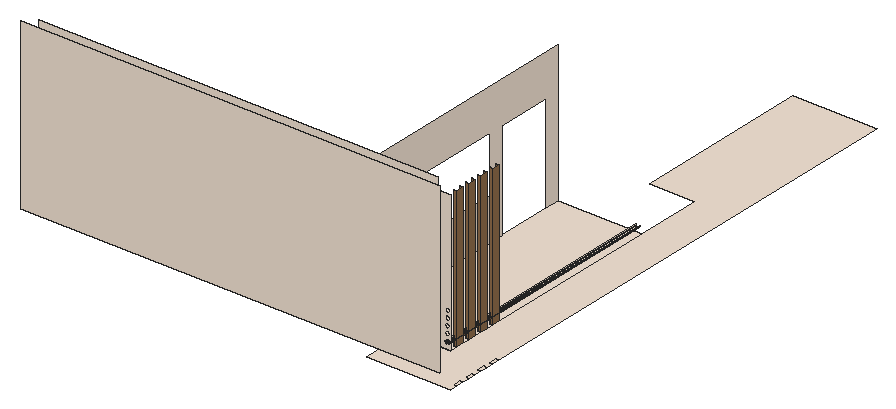
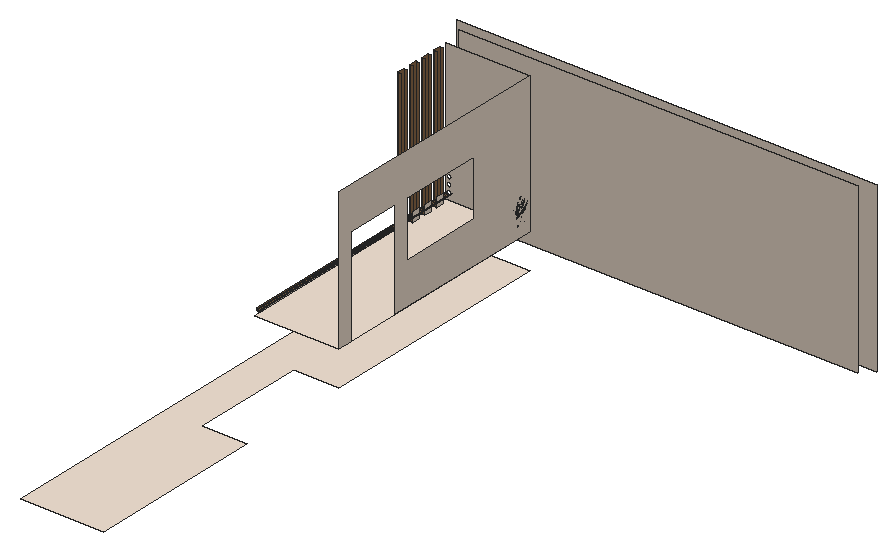
# SketchUp Ruby script. Lengths in inches.
U = 1.inch
M = Sketchup.active_model
def pt(a) = Geom::Point3d.new(a.map { |v| v * U })
def face(e, loops, mat)
  f = e.add_face(loops[0].map { |a| pt(a) })
  loops[1..].each { |l| e.add_face(l.map { |a| pt(a) }).erase! }
  f.material = f.back_material = mat if mat
  f
end
# faces: each face lists its corners as indices into pts; further lists are holes
def faces(e, pts, list, mat = nil) = list.each { |f| face(e, (f[0].is_a?(Array) ? f : [f]).map { |l| l.map { |i| pts[i] } }, mat) }
# xy, xz, yz: faces in a plane at the given z, y or x. An outline is a flat list of corners, or four numbers for a rectangle; further outlines are holes
def ring(l) = l.size == 4 ? [[l[0], l[1]], [l[2], l[1]], [l[2], l[3]], [l[0], l[3]]] : l.each_slice(2).to_a
def flat(e, list, mat, &to3) = list.each { |f| face(e, (f[0].is_a?(Array) ? f : [f]).map { |l| ring(l).map { |u, v| to3.(u, v) } }, mat) }
def xy(e, z, list, mat = nil) = flat(e, list, mat) { |x, y| [x, y, z] }
def xz(e, y, list, mat = nil) = flat(e, list, mat) { |x, z| [x, y, z] }
def yz(e, x, list, mat = nil) = flat(e, list, mat) { |y, z| [x, y, z] }
def lines(e, pts, list) = list.each { |a, b| e.add_line(pt(pts[a]), pt(pts[b])) }
# prism: a flat outline (further loops are holes) pulled along v
def prism(e, loops, v, mat = nil)
  f = face(e, loops, mat); d = Geom::Vector3d.new(v.map { |x| x * U })
  f.pushpull(f.normal.samedirection?(d) ? d.length : -d.length)
end
def box(e, o, s, mat = nil) = prism(e, [[o, [o[0] + s[0], o[1], o[2]], [o[0] + s[0], o[1] + s[1], o[2]], [o[0], o[1] + s[1], o[2]]]], [0, 0, s[2]], mat)
def at(x, y, z, deg = 0) = Geom::Transformation.translation(pt([x, y, z])) * Geom::Transformation.rotation(ORIGIN, Z_AXIS, deg.degrees)
def axes(o, x, y, z) = Geom::Transformation.new([*x, 0, *y, 0, *z, 0, *pt(o).to_a, 1])
def part(name) = M.definitions.add(name)
# library, detail: a bought-in or finely detailed component or shape, given as its bounding box
def library(name, o, s) = part(name).tap { |d| box(d.entities, o, s) }
def detail(e, o, s) = box(e.add_group.entities, o, s)
def put(e, d, t, mat = nil) = e.add_instance(d, t).tap { |i| i.material = mat if mat }
def group(e, t, mat = nil) = e.add_group.tap { |g| g.transformation = t; g.material = mat if mat }.entities
root = M.entities
M.materials.add("C01_Vanilla_Cream").color = [244, 228, 212]
M.materials.add("LightPink_Translucent").color = [144, 107, 117]
M.materials["LightPink_Translucent"].alpha = 0.75
M.materials.add("Wood_Floor_01_1K").color = [146, 111, 76]
c1 = part("blade")
p = [[2.15,0.21,22],[0,0.17,0],[0.09,0.45,0],[2.18,0.31,22],[2.29,0.31,22],[0.38,0.45,0],
  [2.48,0.24,33],[2.49,0.24,33],[2.48,0.22,33]]
faces(c1.entities,p,[[0,1,2,3],[4,5,2,3],[6,3,4,7],[8,0,3,6]])
c2 = part("seeds")
p = [[0.3,-0.1,1.38],[-0.01,-0.03,1.59],[-0.01,-0.03,0.03],[0.14,-0.07,-0.07],[0.29,-0.03,3],[0.15,0.01,3.11]]
faces(c2.entities,p,[[0,1,2,3],[1,0,4,5]],"LightPink_Translucent")
c3 = part("blade with seeds")
put(c3.entities,c1,at(0,0,0))
put(c3.entities,c2,axes([2.4,0.25,30.99],[1.5799,-0.05474,1.17369],[-0.12525,1.92788,0.29478],[-0.07173,-0.02425,1.56792]))
xy(root,132,[[288,12,288,216,326.85,216,326.85,314.71,288,314.71,288,468,360,468,360,63.65,357,63.65,357,57.2,360,57.2,360,50.74,357,50.74,357,44.28,360,44.28,360,37.83,357,37.83,357,31.37,360,31.37,360,24.91,357,24.91,357,18.46,360,18.46,360,12],[357,18.46,360,24.91],[357,31.37,360,37.83],[357,44.28,360,50.74],[357,57.2,360,63.65]],"C01_Vanilla_Cream")
xy(root,162,[[288,12,360,12,360,18.46,357,18.46,357,24.91,360,24.91,360,31.37,357,31.37,357,37.83,360,37.83,360,44.28,357,44.28,357,50.74,360,50.74,360,57.2,357,57.2,357,63.65,360,63.65,360,216,288,216],[357,18.46,360,24.91],[357,31.37,360,37.83],[357,44.28,360,50.74],[357,57.2,360,63.65]],"C01_Vanilla_Cream")
xz(root,0,[[0,150,360,294]],"C01_Vanilla_Cream")
xz(root,9,[[9,150,351,294]],"C01_Vanilla_Cream")
xz(root,12,[[[288,162,360,282],[357,184,357.52,184.07,358,184.27,358.41,184.59,358.73,185,358.93,185.48,359,186,358.93,186.52,358.73,187,358.41,187.41,358,187.73,357.52,187.93,357,188,356.48,187.93,356,187.73,355.59,187.41,355.27,187,355.07,186.52,355,186,355.07,185.48,355.27,185,355.59,184.59,356,184.27,356.48,184.07],[357,190,357.52,190.07,358,190.27,358.41,190.59,358.73,191,358.93,191.48,359,192,358.93,192.52,358.73,193,358.41,193.41,358,193.73,357.52,193.93,357,194,356.48,193.93,356,193.73,355.59,193.41,355.27,193,355.07,192.52,355,192,355.07,191.48,355.27,191,355.59,190.59,356,190.27,356.48,190.07],[357,178,357.52,178.07,358,178.27,358.41,178.59,358.73,179,358.93,179.48,359,180,358.93,180.52,358.73,181,358.41,181.41,358,181.73,357.52,181.93,357,182,356.48,181.93,356,181.73,355.59,181.41,355.27,181,355.07,180.52,355,180,355.07,179.48,355.27,179,355.59,178.59,356,178.27,356.48,178.07],[357,172,357.52,172.07,358,172.27,358.41,172.59,358.73,173,358.93,173.48,359,174,358.93,174.52,358.73,175,358.41,175.41,358,175.73,357.52,175.93,357,176,356.48,175.93,356,175.73,355.59,175.41,355.27,175,355.07,174.52,355,174,355.07,173.48,355.27,173,355.59,172.59,356,172.27,356.48,172.07],[357,166,357.52,166.07,358,166.27,358.41,166.59,358.73,167,358.93,167.48,359,168,358.93,168.52,358.73,169,358.41,169.41,358,169.73,357.52,169.93,357,170,356.48,169.93,356,169.73,355.59,169.41,355.27,169,355.07,168.52,355,168,355.07,167.48,355.27,167,355.59,166.59,356,166.27,356.48,166.07]]],"C01_Vanilla_Cream")
xz(root,18.46,[[357,162,360,282]],"Wood_Floor_01_1K")
xz(root,24.91,[[357,162,360,282]],"Wood_Floor_01_1K")
xz(root,31.37,[[357,162,360,282]],"Wood_Floor_01_1K")
xz(root,37.83,[[357,162,360,282]],"Wood_Floor_01_1K")
xz(root,44.28,[[357,162,360,282]],"Wood_Floor_01_1K")
xz(root,50.74,[[357,162,360,282]],"Wood_Floor_01_1K")
xz(root,57.2,[[357,162,360,282]],"Wood_Floor_01_1K")
xz(root,63.65,[[357,162,360,282]],"Wood_Floor_01_1K")
yz(root,288,[[[12,162,156,162,156,246,204,246,204,162,216,162,216,282,12,282],[72,198,144,246]]],"C01_Vanilla_Cream")
yz(root,357,[[18.46,162,24.91,166],[31.37,162,37.83,166],[44.28,162,50.74,166],[57.2,162,63.65,166],[18.46,166,24.91,170],
  [31.37,166,37.83,170],[44.28,166,50.74,170],[57.2,166,63.65,170]],"C01_Vanilla_Cream")
yz(root,360,[[18.46,162,24.91,282],[31.37,162,37.83,282],[44.28,162,50.74,282],[57.2,162,63.65,282]],"Wood_Floor_01_1K")
p = [[356.48,216,166.07],[357,216,166],[357,63.65,166],[357,57.2,166],[357,50.74,166],[357,44.28,166],
  [357,37.83,166],[357,31.37,166],[357,24.91,166],[357,18.46,166],[357,12,166],[356.48,12,166.07],
  [357.52,216,166.07],[357.52,12,166.07],[356,216,166.27],[356,12,166.27],[358,216,166.27],[358,12,166.27],
  [355.59,216,166.59],[355.59,12,166.59],[358.41,216,166.59],[358.41,12,166.59],[355.27,216,167],[355.27,12,167],
  [358.73,216,167],[358.73,12,167],[355.07,216,167.48],[355.07,12,167.48],[358.93,216,167.48],[358.93,12,167.48],
  [355,216,168],[355,12,168],[359,216,168],[359,12,168]]
faces(root,p,[[0,1,2,3,4,5,6,7,8,9,10,11],[14,0,11,15],[18,14,15,19],[22,18,19,23],[26,22,23,27],[30,26,27,31]],"C01_Vanilla_Cream")
faces(root,p,[[1,12,13,10,9,8,7,6,5,4,3,2],[12,16,17,13],[16,20,21,17],[20,24,25,21],[24,28,29,25],[28,32,33,29]],"Wood_Floor_01_1K")
put(root,c3,axes([295.875,21,164.91],[0.12726,0.15818,1.28532],[-0.58807,0.13317,0.10393],[-0.13291,-0.24832,0.54946]))
put(root,c3,axes([296.85,19.95,165.54],[-0.08515,-0.06907,1.31208],[-0.56828,0.04379,-0.2075],[-0.0907,-0.16522,0.10523]))
put(root,c3,axes([298.17,20.77,163.94],[-0.15825,0.09972,1.07251],[-0.47395,-0.17454,-0.23066],[0.08785,-0.21706,0.45856]))
put(root,c3,axes([297.44,21.12,165.74],[-0.26572,-0.40059,-0.53284],[0.54698,-0.22325,0.0643],[-0.06214,-0.19355,0.75375]))
put(root,c3,axes([295.72,20.58,163.94],[-0.03371,0.16116,1.07251],[-0.49286,0.13491,-0.23066],[-0.11521,-0.20831,0.45856]))
put(root,c3,axes([296.99,20.23,163.12],[-0.09338,0.01775,1.32257],[-0.51641,-0.1998,-0.20205],[0.00867,-0.16666,0.22528]))
put(root,c3,axes([298.55,21.51,165.74],[0.01449,-0.45571,-0.53284],[0.61002,0.03061,0.0643],[0.06438,-0.19306,0.75375]))
put(root,c3,axes([299.4,20.8,165.54],[-0.00537,-0.09805,1.31208],[-0.45391,-0.28338,-0.2075],[0.07018,-0.17178,0.10523]))
put(root,c3,axes([297.49,20.78,165.39],[0.16784,-0.37886,-0.2656],[0.48968,0.1105,0.3429],[-0.0449,-0.15254,0.65611]))
put(root,c3,axes([297.86,21.28,164.91],[-0.10366,0.16934,1.28532],[-0.43488,-0.35044,0.10393],[0.19618,-0.21841,0.54946]))
put(root,c3,axes([299.28,20.44,165.53],[-0.05654,0.03763,1.33037],[-0.55396,-0.12696,-0.12571],[-0.02005,-0.16422,0.23543]))
put(root,c3,axes([297.24,21.04,165.51],[-0.54728,-0.1235,-0.38324],[0.18759,-0.42344,-0.29685],[-0.05018,-0.17048,0.7333]))
put(root,c3,axes([297.58,19.98,164.07],[0.07142,0.28728,0.86145],[-0.3962,-0.15911,0.63294],[0.04263,-0.1471,0.18974]))
put(root,c3,axes([298.43,21.36,165.51],[-0.39855,-0.33102,-0.38324],[0.42102,-0.2899,-0.29685],[0.06064,-0.16819,0.7333]))
put(root,c3,axes([296.26,19.72,165.53],[-0.01039,0.05905,1.33037],[-0.51226,0.21431,-0.12571],[-0.15074,-0.10955,0.23543]))
put(root,c3,axes([296.15,20.77,165.82],[0.62019,-0.12663,0.40322],[0.10763,0.49673,0.33247],[-0.14586,-0.1464,0.83437]))
put(root,c3,axes([297.55,20.86,165.55],[0.54859,0.1288,0.36002],[-0.18759,0.42344,0.29685],[-0.03297,-0.16652,0.74497]))
put(root,c3,axes([297.71,21.02,165.78],[-0.54481,0.22937,-0.0912],[-0.26773,-0.4071,-0.50621],[-0.07188,-0.17155,0.76918]))
put(root,c3,axes([298.84,21.53,165.78],[-0.61188,-0.02441,-0.0912],[0.01672,-0.46217,-0.50621],[0.0425,-0.178,0.76918]))
put(root,c3,axes([298.8,21.23,165.39],[0.3767,-0.25939,-0.2656],[0.3566,0.29618,0.3429],[0.05426,-0.15048,0.65611]))
put(root,c3,axes([295.55,20.32,164.07],[0.29042,0.17147,0.86145],[-0.42295,0.10307,0.63294],[-0.0905,-0.13178,0.18974]))
put(root,c3,axes([297.7,20.83,165.55],[0.41024,-0.16744,0.04823],[0.2008,0.30532,0.37966],[-0.03962,-0.13459,0.57892]))
put(root,c3,axes([296.25,21.23,165.74],[-0.47473,-0.23813,-0.53284],[0.33738,-0.41728,0.0643],[-0.172,-0.14218,0.75375]))
put(root,c3,axes([296.08,20.91,165.39],[-0.08599,-0.39682,-0.2656],[0.49155,-0.10478,0.3429],[-0.13203,-0.11372,0.65611]))
put(root,c3,axes([296.29,20.88,165.55],[0.25304,-0.31296,0.04823],[0.36033,0.18221,0.37966],[-0.11649,-0.10034,0.57892]))
put(root,c3,axes([295.32,20.84,163.12],[-0.05393,0.0649,1.32257],[-0.545,0.13993,-0.20205],[-0.13166,-0.12729,0.22528]))
put(root,c3,axes([296.22,22.62,163.57],[-0.22864,-0.5052,-0.52377],[0.65862,-0.18195,-0.13747],[-0.02527,-0.17107,1.15612]))
put(root,c3,axes([295.02,21.49,164.91],[0.2068,0.08488,1.28532],[-0.42797,0.35609,0.10393],[-0.26673,-0.16064,0.54946]))
put(root,c3,axes([299.27,21.08,163.12],[-0.08333,-0.03881,1.32257],[-0.21404,-0.4336,-0.20205],[0.14439,-0.11767,0.22528]))
put(root,c3,axes([297.55,21.17,165.79],[-0.16784,0.37886,0.2656],[-0.48968,-0.1105,-0.3429],[-0.0449,-0.15254,0.65611]))
put(root,c3,axes([296.02,21.24,165.51],[-0.54938,0.11711,-0.38324],[-0.0961,-0.44351,-0.29685],[-0.14756,-0.1271,0.7333]))
put(root,c3,axes([298.8,21.33,165.55],[0.39645,0.33614,0.36002],[-0.42102,0.2899,0.29685],[0.07313,-0.15771,0.74497]))
put(root,c3,axes([296.41,20.85,166.07],[-0.37157,0.4723,-0.10215],[-0.5381,-0.2721,-0.56695],[-0.18705,-0.13344,0.86148]))
put(root,c3,axes([298.95,21.37,165.55],[0.45752,0.02296,0.04823],[-0.01254,0.34663,0.37966],[0.04787,-0.13278,0.57892]))
put(root,c3,axes([298.6,21.6,165.79],[-0.3767,0.25939,0.2656],[-0.3566,-0.29618,-0.3429],[0.05426,-0.15048,0.65611]))
put(root,c3,axes([299.27,22.3,165.74],[0.29081,-0.38873,-0.53284],[0.5096,0.27626,0.0643],[0.17364,-0.14084,0.75375]))
put(root,c3,axes([296.125,21.17,163.78],[-0.34808,-0.49367,0],[0.58235,-0.27531,-0.38706],[0.13264,-0.0627,1.22783]))
put(root,c3,axes([299.25,22.12,165.51],[-0.14302,-0.44985,-0.38324],[0.54163,-0.07869,-0.29685],[0.15522,-0.12083,0.7333]))
put(root,c3,axes([296.89,20.57,163.6],[-0.38473,0.28263,-0.02919],[-0.35252,-0.30954,-0.13237],[-0.02482,-0.08771,0.43661]))
put(root,c3,axes([294.98,20.71,165.54],[-0.11979,-0.00348,1.31208],[-0.38137,0.34775,-0.2075],[-0.20349,-0.07106,0.10523]))
put(root,c3,axes([299.51,22.44,165.78],[-0.515,-0.27165,-0.0912],[0.2967,-0.3934,-0.50621],[0.1455,-0.13675,0.76918]))
put(root,c3,axes([297.38,23.92,164.49],[0.48111,0.19866,1.13446],[-0.47133,0.42798,0.44862],[-0.21112,-0.25366,0.95105]))
put(root,c3,axes([296.37,21.24,165.79],[0.08599,0.39682,0.2656],[-0.49155,0.10478,-0.3429],[-0.13203,-0.11372,0.65611]))
put(root,c3,axes([294.87,22.55,163.51],[0,-0.49266,-0.37238],[0.62289,0,0],[0,-0.11221,1.18128]))
put(root,c3,axes([296.6,21.09,163.51],[0.52105,-0.24633,-0.37238],[0.31144,0.44171,0],[0.11867,-0.0561,1.18128]))
put(root,c3,axes([299.69,21.94,163.94],[-0.19889,-0.01459,1.07251],[-0.20376,-0.39145,-0.23066],[0.24434,-0.11074,0.45856]))
put(root,c3,axes([294.9,21.5,165.82],[0.45978,-0.36358,0.40322],[0.39653,0.38611,0.33247],[-0.21571,-0.06707,0.83437]))
put(root,c3,axes([300.78,22.32,165.53],[-0.07272,-0.00374,1.33037],[-0.30197,-0.40092,-0.12571],[0.12127,-0.13182,0.23543]))
put(root,c3,axes([297.22,22.1,163.54],[0.375,-0.3703,-0.46765],[0.46584,0.33578,-0.12274],[0.15027,-0.09237,1.03225]))
put(root,c3,axes([299.92,21.22,164.07],[-0.18544,0.25079,0.86145],[-0.15939,-0.33694,0.63294],[0.15316,-0.08443,0.18974]))
put(root,c3,axes([299.65,22.17,165.39],[0.48462,-0.07041,-0.2656],[0.12797,0.4025,0.3429],[0.13888,-0.10811,0.65611]))
put(root,c3,axes([295.11,21.49,165.55],[0.02803,-0.37463,0.04823],[0.42332,0.01027,0.37966],[-0.16216,-0.0392,0.57892]))
put(root,c3,axes([296.5625,22.75,163.66],[0.27012,-0.44393,-0.33554],[0.56127,0.21365,0.16149],[0,-0.10233,1.07733]))
put(root,c3,axes([294.94,21.61,165.39],[-0.31678,-0.30846,-0.2656],[0.36171,-0.29199,0.3429],[-0.18378,-0.04443,0.65611]))
put(root,c3,axes([296.81,22.53,164],[-0.06488,-0.56215,-0.21822],[0.6757,-0.03399,-0.37502],[0.11898,-0.07488,1.19781]))
put(root,c3,axes([295.13,22.5625,163.52],[0.38863,-0.30738,-0.23233],[0.38863,0.30738,0.23233],[0,-0.09901,1.0423]))
put(root,c3,axes([294.98,21.09,163.6],[-0.1606,0.40228,-0.02919],[-0.4943,-0.12375,-0.13237],[-0.07505,-0.0658,0.43661]))
put(root,c3,axes([299.26,22.4,165.79],[-0.48462,0.07041,0.2656],[-0.12797,-0.4025,-0.3429],[0.13888,-0.10811,0.65611]))
put(root,c3,axes([296.5,23.12,164],[-0.62699,-0.23507,-0.21822],[0.3019,-0.49615,-0.37502],[-0.0197,-0.12182,1.19781]))
put(root,c3,axes([294.71,22.92,163.78],[-0.69617,0,0],[0,-0.55062,-0.38706],[0,-0.12541,1.22783]))
put(root,c3,axes([294.83,21.94,163.94],[0.1087,0.13716,1.07251],[-0.25048,0.37284,-0.23066],[-0.25719,-0.08912,0.45856]))
put(root,c3,axes([296.72,21.29,163.52],[0.51941,0.1219,-0.23233],[-0.13078,0.42928,0.23233],[0.10471,-0.0495,1.0423]))
put(root,c3,axes([295.28,21.82,165.74],[-0.55654,-0.01186,-0.53284],[0.03738,-0.49951,0.0643],[-0.23578,-0.05271,0.75375]))
put(root,c3,axes([299.7,22.34,165.55],[0.3822,0.20719,0.04823],[-0.22252,0.29505,0.37966],[0.12254,-0.09539,0.57892]))
put(root,c3,axes([299.59,22.25,165.55],[0.13808,0.45342,0.36002],[-0.54163,0.07869,0.29685],[0.15963,-0.10664,0.74497]))
put(root,c3,axes([301.05,22.8,165.54],[0.07726,-0.07504,1.31208],[-0.09888,-0.46032,-0.2075],[0.19384,-0.08728,0.10523]))
put(root,c3,axes([295.25,22.78,163.75],[-0.51786,0.4142,0.23067],[-0.51817,-0.40984,-0.27369],[-0.01808,-0.11762,1.23664]))
put(root,c3,axes([294.52,21,165.53],[0.04127,0.04917,1.33037],[-0.19898,0.44196,-0.12571],[-0.20151,0.0032,0.23543]))
put(root,c3,axes([296.9,22.97,163.82],[0.6273,0.23878,0.18048],[-0.3019,0.49615,0.37502],[0,-0.11437,1.20407]))
put(root,c3,axes([296.65,23.64,163.83],[0.14756,-0.58378,-0.17572],[0.69966,0.10176,0.38453],[-0.12225,-0.08062,1.1733]))
put(root,c3,axes([295.09,21.92,165.51],[-0.40426,0.32635,-0.38324],[-0.35404,-0.34474,-0.29685],[-0.2054,-0.04965,0.7333]))
put(root,c3,axes([295.39,21.77,165.79],[0.31678,0.30846,0.2656],[-0.36171,0.29199,-0.3429],[-0.18378,-0.04443,0.65611]))
put(root,c3,axes([294.18,22.35,164.07],[0.35544,-0.03525,0.86145],[-0.22547,0.31061,0.63294],[-0.17565,-0.04659,0.18974]))
put(root,c3,axes([296.7,22.64,164.04],[-0.60457,0.03041,0.33554],[-0.05467,-0.50484,-0.16149],[0.10823,-0.05117,1.07733]))
put(root,c3,axes([295.31,21.58,165.78],[-0.02981,0.50103,-0.0912],[-0.56442,-0.01369,-0.50621],[-0.21738,-0.0348,0.76918]))
put(root,c3,axes([295.13,23.01,163.86],[0,0.49266,0.37238],[-0.62289,0,0],[0,-0.11221,1.18128]))
put(root,c3,axes([299.53,23.5,165.78],[-0.28012,-0.44611,-0.0912],[0.49717,-0.21923,-0.50621],[0.20951,-0.05886,0.76918]))
put(root,c3,axes([299.51,23.12,165.51],[0.15083,-0.44814,-0.38324],[0.51712,0.15361,-0.29685],[0.2082,-0.04109,0.7333]))
put(root,c3,axes([298.6875,21.29,163.78],[0.34808,-0.49367,0],[0.58235,0.27531,-0.38706],[0.13264,0.0627,1.22783]))
put(root,c3,axes([294.59,22.27,164.91],[0.23093,-0.01116,1.28532],[-0.15319,0.4836,0.10393],[-0.32909,-0.02991,0.54946]))
put(root,c3,axes([296.6,23.4,163.66],[-0.33445,-0.41351,-0.33554],[0.50659,-0.29119,0.16149],[-0.10823,-0.05117,1.07733]))
put(root,c3,axes([296.67,22.82,163.77],[0.24206,0.5509,0.34316],[-0.69162,0.19157,0.13466],[0.00845,-0.10123,1.19142]))
put(root,c3,axes([300.06,23.24,163.49],[-0.35858,0.05912,1.06187],[-0.05708,-0.47061,0.06078],[0.25115,-0.07123,0.60425]))
put(root,c3,axes([300.71,22.83,163.7],[-0.34516,-0.31503,-0.04866],[0.37803,-0.28865,-0.22062],[0.10711,-0.02032,0.72768]))
put(root,c3,axes([296.55,23.25,164.04],[-0.27012,0.44393,0.33554],[-0.56127,-0.21365,-0.16149],[0,-0.10233,1.07733]))
put(root,c3,axes([297.54,22.87,163.65],[0,-0.57005,0],[0.69617,0,0],[0,0,1.34592]))
put(root,c3,axes([298.39,21.55,163.86],[-0.52105,-0.24633,0.37238],[0.31144,-0.44171,0],[0.11867,0.0561,1.18128]))
put(root,c3,axes([299.41,23.28,165.74],[0.48922,-0.21758,-0.53284],[0.27264,0.44789,0.0643],[0.23638,-0.05088,0.75375]))
put(root,c3,axes([296.3,23.5625,163.54],[-0.57914,-0.08077,-0.46765],[0.12221,-0.49823,-0.12274],[-0.17283,-0.06037,1.03225]))
put(root,c3,axes([297.21,22.51,163.77],[-0.46162,0.4471,0.34316],[-0.54842,-0.39467,0.13466],[0.11129,-0.04462,1.19142]))
put(root,c3,axes([297.72,23.31,163.72],[-0.51786,-0.42404,-0.04598],[0.51817,-0.4243,0],[-0.01808,-0.01481,1.31678]))
put(root,c3,axes([296.41,21.77,163.86],[-0.16083,0.48962,0.13232],[-0.58854,-0.13856,0.26315],[0.10167,-0.00238,1.20305]))
put(root,c3,axes([299.34,23.37,165.79],[-0.46269,-0.13744,0.2656],[0.13495,-0.40096,-0.3429],[0.18628,-0.03677,0.65611]))
put(root,c3,axes([294.49,22.63,165.55],[0.15729,-0.44921,0.36002],[0.51712,0.15361,0.29685],[-0.20336,0.027,0.74497]))
put(root,c3,axes([296.17,22.17,163.2],[-0.548,0.19724,0.96696],[-0.17442,-0.56594,0.37572],[0.3365,0.00941,1.09981]))
put(root,c3,axes([297.64,22.32,163.96],[0.1074,-0.43968,0.1086],[0.52474,0.07632,-0.3101],[0.0955,0.04515,0.95058]))
put(root,c3,axes([294.45,22.51,165.55],[-0.20448,-0.33592,0.04823],[0.37288,-0.16442,0.37966],[-0.16437,0.03244,0.57892]))
put(root,c3,axes([296.73,23.36,163.77],[0.70367,0.1038,0.34316],[-0.1432,0.58624,0.13466],[-0.10283,-0.05661,1.19142]))
put(root,c3,axes([300.45,22.9375,163.12],[-0.0291,-0.0748,1.32257],[0.20181,-0.43752,-0.20205],[0.20357,-0.00629,0.22528]))
put(root,c3,axes([294.44,22.86,163.12],[0.01412,0.07764,1.32257],[-0.28464,0.40547,-0.20205],[-0.20218,-0.02044,0.22528]))
put(root,c3,axes([297.42,22.43,164.04],[-0.33445,-0.41351,0.33554],[0.50659,-0.29119,-0.16149],[0.10823,0.05117,1.07733]))
put(root,c3,axes([295.6875,24.32,163.52],[-0.13078,-0.42928,-0.23233],[0.51941,-0.1219,0.23233],[-0.10471,-0.0495,1.0423]))
put(root,c3,axes([296.36,24.3,163.86],[0.59825,-0.13076,0.13232],[0.14773,0.48663,0.26315],[-0.05336,-0.0709,1.20305]))
put(root,c3,axes([297.59,22.46,164],[0.56211,-0.32708,-0.21822],[0.3738,0.46216,-0.37502],[0.13869,0.04694,1.19781]))
put(root,c3,axes([299.82,23.32,165.39],[0.46269,0.13744,-0.2656],[-0.13495,0.40096,0.3429],[0.18628,-0.03677,0.65611]))
put(root,c3,axes([295.54,24.51,163.51],[-0.52105,-0.24633,-0.37238],[0.31144,-0.44171,0],[-0.11867,-0.0561,1.18128]))
put(root,c3,axes([299.01,21.59,163.51],[0.52105,0.24633,-0.37238],[-0.31144,0.44171,0],[0.11867,0.0561,1.18128]))
put(root,c3,axes([294.38,22.68,165.39],[-0.46269,-0.13744,-0.2656],[0.13495,-0.40096,0.3429],[-0.18628,0.03677,0.65611]))
put(root,c3,axes([298.02,23,163.65],[0.62289,0,0],[0,0.51004,0],[0,0,1.33805]))
put(root,c3,axes([296.96,23.64,164],[-0.56211,0.32708,-0.21822],[-0.3738,-0.46216,-0.37502],[-0.13869,-0.04694,1.19781]))
put(root,c3,axes([298.19,21.8,163.86],[-0.59825,0.13076,0.13232],[-0.14773,-0.48663,0.26315],[0.05336,0.0709,1.20305]))
put(root,c3,axes([298.5625,22.83,164.91],[-0.23093,0.01116,1.28532],[0.15319,-0.4836,0.10393],[0.32909,0.02991,0.54946]))
put(root,c3,axes([298.86,21.77,163.52],[0.13078,0.42928,-0.23233],[-0.51941,0.1219,0.23233],[0.10471,0.0495,1.0423]))
put(root,c3,axes([299.76,23.49,165.55],[0.20448,0.33592,0.04823],[-0.37288,0.16442,0.37966],[0.16437,-0.03244,0.57892]))
put(root,c3,axes([297.82,22.74,163.79],[-0.70367,-0.1038,0.36899],[0.1432,-0.58624,0.1448],[0.10283,0.05661,1.2811]))
put(root,c3,axes([299.72,23.37,165.55],[-0.15729,0.44921,0.36002],[-0.51712,-0.15361,0.29685],[0.20336,-0.027,0.74497]))
put(root,c3,axes([297.25,24.18,163.65],[-0.18165,-0.42474,0],[0.51872,-0.14874,0],[0,0,1.15778]))
put(root,c3,axes([296.91,23.78,163.96],[-0.1074,0.43968,0.1086],[-0.52474,-0.07632,-0.3101],[-0.0955,-0.04515,0.95058]))
put(root,c3,axes([294.87,22.64,165.79],[0.46269,0.13744,0.2656],[-0.13495,0.40096,-0.3429],[-0.18628,0.03677,0.65611]))
put(root,c3,axes([297.93,24.125,163.64],[0.5845,-0.16716,-0.14398],[0.20539,0.48152,0.00006],[0.06452,-0.01848,1.30423]))
put(root,c3,axes([298.14,24.32,163.86],[0.16083,-0.48962,0.13232],[0.58854,0.13856,0.26315],[-0.10167,0.00238,1.20305]))
put(root,c3,axes([298,23.21,163.66],[0.38863,0.31822,0],[-0.38863,0.31822,0],[0,0,1.2695]))
put(root,c3,axes([295.79,22.62,164.51],[0.15825,-0.07127,1.32798],[0.05457,0.4976,0.10393],[-0.34278,0.06603,0.47463]))
put(root,c3,axes([299.06,23.07,163.86],[-0.43742,-0.35886,0.13232],[0.44081,-0.34807,0.26315],[-0.04831,0.07329,1.20305]))
put(root,c3,axes([298.25,22.53,163.54],[0.57914,0.08077,-0.46765],[-0.12221,0.49823,-0.12274],[0.17283,0.06037,1.03225]))
put(root,c3,axes([300.8,23.4,164.07],[-0.34399,0.08133,0.86145],[0.16192,-0.33614,0.63294],[0.18249,0.023,0.18974]))
put(root,c3,axes([297.125,24.375,163.65],[-0.56127,-0.22118,0],[0.27012,-0.45959,0],[0,0,1.2203]))
put(root,c3,axes([297.59,23.79,163.85],[-0.54364,-0.39653,-0.18894],[0.45745,-0.44527,0.41347],[-0.14639,0.04639,1.26162]))
put(root,c3,axes([296.16,24.55,163.86],[0.52105,0.24633,0.37238],[-0.31144,0.44171,0],[-0.11867,-0.0561,1.18128]))
put(root,c3,axes([298,22.84,164.04],[0.27012,-0.44393,0.33554],[0.56127,0.21365,-0.16149],[0,0.10233,1.07733]))
put(root,c3,axes([300.65,24.83,165.53],[-0.05034,-0.04313,1.33037],[0.11012,-0.46232,-0.12571],[0.1983,-0.02954,0.23543]))
put(root,c3,axes([294.09,22.95,165.54],[-0.09091,0.06396,1.31208],[0.00773,0.46734,-0.2075],[-0.20839,0.06078,0.10523]))
put(root,c3,axes([297.89,23.1,163.72],[0,0.56976,-0.04228],[-0.69617,0,0],[0,0.01791,1.34526]))
put(root,c3,axes([294.7,22.89,165.51],[-0.15083,0.44814,-0.38324],[-0.51712,-0.15361,-0.29685],[-0.2082,0.04109,0.7333]))
put(root,c3,axes([294.68,22.5,165.78],[0.28012,0.44611,-0.0912],[-0.49717,0.21923,-0.50621],[-0.20951,0.05886,0.76918]))
put(root,c3,axes([297.95,22.69,163.66],[0.33445,0.41351,-0.33554],[-0.50659,0.29119,0.16149],[0.10823,0.05117,1.07733]))
put(root,c3,axes([300.21,24.44,164.95],[-0.10656,-0.41414,-0.02619],[0.50364,-0.09521,-0.11874],[0.10517,0.02626,0.39164]))
put(root,c3,axes([295.86,24.8,163.78],[-0.34808,0.49367,0],[-0.58235,-0.27531,-0.38706],[-0.13264,-0.0627,1.22783]))
put(root,c3,axes([298.9,24.43,165.78],[0.02981,-0.50103,-0.0912],[0.56442,0.01369,-0.50621],[0.21738,0.0348,0.76918]))
put(root,c3,axes([299.42,23.09,163.86],[0,-0.49266,0.37238],[0.62289,0,0],[0,0.11221,1.18128]))
put(root,c3,axes([297.86,23.46,164.04],[0.60457,-0.03041,0.33554],[0.05467,0.50484,-0.16149],[-0.10823,0.05117,1.07733]))
put(root,c3,axes([298.23,22.94,163.96],[0.51872,-0.14368,0.1086],[0.18165,0.41027,-0.3101],[0,0.09029,0.95058]))
put(root,c3,axes([298.81,24.23,165.79],[-0.31678,-0.30846,0.2656],[0.36171,-0.29199,-0.3429],[0.18378,0.04443,0.65611]))
put(root,c3,axes([297.32,23.7,163.66],[-0.60457,0.03041,-0.33554],[-0.05467,-0.50484,0.16149],[-0.10823,0.05117,1.07733]))
put(root,c3,axes([300.16,23.94,163.94],[-0.13408,-0.12117,1.07251],[0.17446,-0.40083,-0.23066],[0.27128,0.0543,0.45856]))
put(root,c3,axes([297.76,24.38,163.65],[0.56127,0.22118,0],[-0.27012,0.45959,0],[0,0,1.31215]))
put(root,c3,axes([299.39,24.125,165.54],[0.11943,-0.00833,1.31208],[0.32759,-0.38275,-0.2075],[0.21244,0.05052,0.10523]))
put(root,c3,axes([297.99,24.87,163.64],[-0.34375,-0.4954,-0.03857],[0.58235,-0.27531,0.38706],[-0.1435,0.04717,1.22723]))
put(root,c3,axes([297.87,23.67,163.96],[0.41131,0.296,0.1086],[-0.34309,0.33395,-0.3101],[-0.0955,0.04515,0.95058]))
put(root,c3,axes([294.62,23.75,165.55],[-0.13808,-0.45342,0.36002],[0.54163,-0.07869,0.29685],[-0.15963,0.10664,0.74497]))
put(root,c3,axes([294.51,23.66,165.55],[-0.3822,-0.20719,0.04823],[0.22252,-0.29505,0.37966],[-0.12254,0.09539,0.57892]))
put(root,c3,axes([294.68,23.12,164.91],[0.19317,-0.10421,1.28532],[0.16263,0.48153,0.10393],[-0.30326,0.10883,0.54946]))
put(root,c3,axes([298.93,24.1875,165.74],[0.55654,0.01186,-0.53284],[-0.03738,0.49951,0.0643],[0.23578,0.05271,0.75375]))
put(root,c3,axes([298.3,24.59,163.86],[0.52105,-0.24633,0.37238],[0.31144,0.44171,0],[-0.11867,0.0561,1.18128]))
put(root,c3,axes([297.5625,24.2,163.72],[0.24206,0.56598,-0.04509],[-0.69162,0.19832,0],[0.00845,0.01976,1.2913]))
put(root,c3,axes([297.83,24.81,163.52],[-0.51941,-0.1219,-0.23233],[0.13078,-0.42928,0.23233],[-0.10471,0.0495,1.0423]))
put(root,c3,axes([294.08,23.9375,163.94],[0.19348,0.04044,1.07251],[0.1247,0.41309,-0.23066],[-0.26282,0.07733,0.45856]))
put(root,c3,axes([294.95,23.6,165.79],[0.48462,-0.07041,0.2656],[0.12797,0.4025,-0.3429],[-0.13888,0.10811,0.65611]))
put(root,c3,axes([299.84,23.17,163.78],[0.69617,0,0],[0,0.55062,-0.38706],[0,0.12541,1.22783]))
put(root,c3,axes([293.08,23.42,165.53],[0.07105,0.01321,1.33037],[0.2198,0.43529,-0.12571],[-0.14545,0.11425,0.23543]))
put(root,c3,axes([299.5625,23.46,163.65],[-0.69582,-0.00394,-0.03732],[0,-0.55062,0.37457],[-0.02187,0.12535,1.18764]))
put(root,c3,axes([298.05,22.98,164],[0.62699,0.23507,-0.21822],[-0.3019,0.49615,-0.37502],[0.0197,0.12182,1.19781]))
put(root,c3,axes([293.68,24.8,164.07],[0.23202,-0.22328,0.86145],[0.09155,0.35348,0.63294],[-0.16768,0.06329,0.18974]))
put(root,c3,axes([299.26,24.39,165.39],[0.31678,0.30846,-0.2656],[-0.36171,0.29199,0.3429],[0.18378,0.04443,0.65611]))
put(root,c3,axes([299.42,23.54,163.52],[-0.38863,0.30738,-0.23233],[-0.38863,-0.30738,0.23233],[0,0.09901,1.0423]))
put(root,c3,axes([297.74,23.57,164],[0.06488,0.56215,-0.21822],[-0.6757,0.03399,-0.37502],[-0.11898,0.07488,1.19781]))
put(root,c3,axes([299.1,24.51,165.55],[-0.02803,0.37463,0.04823],[-0.42332,-0.01027,0.37966],[0.16216,0.0392,0.57892]))
put(root,c3,axes([297.99,23.35,163.66],[-0.27012,0.44393,-0.33554],[-0.56127,-0.21365,0.16149],[0,0.10233,1.07733]))
put(root,c3,axes([294.55,23.84,165.39],[-0.48462,0.07041,-0.2656],[-0.12797,-0.4025,0.3429],[-0.13888,0.10811,0.65611]))
put(root,c3,axes([299.14,24.39,165.55],[-0.41051,0.32462,0.36002],[-0.35404,-0.34474,0.29685],[0.1926,0.05988,0.74497]))
put(root,c3,axes([293.85,24.74,166.23],[0.49129,0.13151,-0.04866],[-0.15113,0.40475,-0.22062],[-0.08035,0.06145,0.72768]))
put(root,c3,axes([297.33,23.99,163.54],[-0.375,0.3703,-0.46765],[-0.46584,-0.33578,-0.12274],[-0.15027,0.09237,1.03225]))
put(root,c3,axes([297.84,24.77,165.79],[-0.08599,-0.39682,0.2656],[0.49155,-0.10478,-0.3429],[0.13203,0.11372,0.65611]))
put(root,c3,axes([298,24.62,163.75],[0.697,0.16013,0.23067],[-0.17437,0.57237,-0.27369],[-0.11536,0.07164,1.23664]))
put(root,c3,axes([297.95,25,163.51],[-0.52105,0.24633,-0.37238],[-0.31144,-0.44171,0],[-0.11867,0.0561,1.18128]))
put(root,c3,axes([299.68,23.55,163.51],[0,0.49266,-0.37238],[-0.62289,0,0],[0,0.11221,1.18128]))
put(root,c3,axes([298.125,23.6,164.91],[-0.2068,-0.08488,1.28532],[0.42797,-0.35609,0.10393],[0.26673,0.16064,0.54946]))
put(root,c3,axes([298.17,22.48,165.36],[-0.48108,-0.25598,1.03712],[0.50798,-0.39855,0.44749],[0.15521,0.24018,1.00248]))
put(root,c3,axes([294.7,23.5625,165.78],[0.515,0.27165,-0.0912],[-0.2967,0.3934,-0.50621],[-0.1455,0.13675,0.76918]))
put(root,c3,axes([298.89,24.57,164.07],[-0.31347,-0.14166,0.86145],[0.40476,-0.14393,0.63294],[0.10917,0.12192,0.18974]))
put(root,c3,axes([297.79,24.97,165.78],[0.33176,-0.4217,-0.0912],[0.48044,0.24295,-0.50621],[0.16701,0.11914,0.76918]))
put(root,c3,axes([295.39,23.44,164.91],[0.13906,-0.15138,1.28532],[0.35111,0.40859,0.10393],[-0.24082,0.18608,0.54946]))
put(root,c3,axes([294.95,23.89,165.51],[0.14302,0.44985,-0.38324],[-0.54163,0.07869,-0.29685],[-0.15522,0.12083,0.7333]))
put(root,c3,axes([295.6,24.4,165.79],[0.3767,-0.25939,0.2656],[0.3566,0.29618,-0.3429],[-0.05426,0.15048,0.65611]))
put(root,c3,axes([298.43,24.93,163.78],[0.34808,0.49367,0],[-0.58235,0.27531,-0.38706],[-0.13264,0.0627,1.22783]))
put(root,c3,axes([297.36,25.32,165.53],[0.00165,-0.05965,1.33037],[0.47711,-0.26315,-0.12571],[0.16572,0.09393,0.23543]))
put(root,c3,axes([298.98,25.09,163.12],[0.04056,-0.07113,1.32257],[0.51066,-0.20948,-0.20205],[0.15482,0.10842,0.22528]))
put(root,c3,axes([298.13,22.97,164.13],[-0.01521,-0.46386,1.05954],[0.68831,0.12024,0.44862],[-0.1628,0.25382,1.00012]))
put(root,c3,axes([298.31,23.48,163.57],[0.20414,0.45107,-0.51909],[-0.58805,0.16245,-0.13624],[0.02256,0.15274,1.1458]))
put(root,c3,axes([295.26,24.64,165.55],[-0.45752,-0.02296,0.04823],[0.01254,-0.34663,0.37966],[-0.04787,0.13278,0.57892]))
put(root,c3,axes([294.29,25.03,163.12],[0.07468,0.04922,1.32257],[0.12663,0.45605,-0.20205],[-0.16551,0.09725,0.22528]))
put(root,c3,axes([295.41,24.67,165.55],[-0.39645,-0.33614,0.36002],[0.42102,-0.2899,0.29685],[-0.07313,0.15771,0.74497]))
put(root,c3,axes([298.18,24.76,165.51],[0.54938,-0.11711,-0.38324],[0.0961,0.44351,-0.29685],[0.14756,0.1271,0.7333]))
put(root,c3,axes([296.66,24.83,165.79],[0.16784,-0.37886,0.2656],[0.48968,0.1105,-0.3429],[0.0449,0.15254,0.65611]))
put(root,c3,axes([298.94,25.21,164],[-0.35702,-0.01545,0.78795],[0.23577,-0.32816,0.43504],[0.14104,0.11659,0.61808]))
put(root,c3,axes([297.91,25.125,165.55],[-0.25304,0.31296,0.04823],[-0.36033,-0.18221,0.37966],[0.11649,0.10034,0.57892]))
put(root,c3,axes([297.32,26.18,166.23],[0.38473,-0.28263,-0.04866],[0.35252,0.30954,-0.22062],[0.02482,0.08771,0.72768]))
put(root,c3,axes([298.02,25.04,165.55],[-0.55374,0.11306,0.36002],[-0.0961,-0.44351,0.29685],[0.13023,0.13071,0.74497]))
put(root,c3,axes([295.29,23.82,164.91],[0.10366,-0.16934,1.28532],[0.43488,0.35044,0.10393],[-0.19618,0.21841,0.54946]))
put(root,c3,axes([297.78,24.42,163.94],[0.00982,-0.16331,1.07251],[0.4695,-0.18242,-0.23066],[0.14493,0.19547,0.45856]))
put(root,c3,axes([296.51,25.17,165.55],[-0.41024,0.16744,0.04823],[-0.2008,-0.30532,0.37966],[0.03962,0.13459,0.57892]))
put(root,c3,axes([295.41,24.77,165.39],[-0.3767,0.25939,-0.2656],[-0.3566,-0.29618,0.3429],[-0.05426,0.15048,0.65611]))
put(root,c3,axes([294.11,24.69,165.54],[-0.01384,0.09749,1.31208],[0.39274,0.33916,-0.2075],[-0.10282,0.16039,0.10523]))
put(root,c3,axes([295.36,24.47,166.05],[0.61188,0.02441,-0.10123],[-0.01672,0.46217,-0.56189],[-0.0425,0.178,0.85379]))
put(root,c3,axes([296.5,24.99,165.78],[0.54481,-0.22937,-0.0912],[0.26773,0.4071,-0.50621],[0.07188,0.17155,0.76918]))
put(root,c3,axes([296.65,25.14,165.8],[-0.54859,-0.1288,0.39962],[0.18759,-0.42344,0.32951],[0.03297,0.16652,0.82692]))
put(root,c3,axes([295.65,25.78,164.07],[-0.01441,-0.29294,0.86145],[0.36003,0.20894,0.63294],[-0.07081,0.13963,0.18974]))
put(root,c3,axes([296.59,25.08,163.12],[0.0901,-0.02681,1.32257],[0.54199,0.14755,-0.20205],[0.01585,0.1663,0.22528]))
put(root,c3,axes([295.78,24.65,165.75],[0.39855,0.33102,-0.4254],[-0.42102,0.2899,-0.32951],[-0.06064,0.16819,0.81396]))
put(root,c3,axes([295.35,25.15,164.12],[0.50577,-0.08724,0.04881],[0.11627,0.35148,-0.64728],[-0.03206,0.17792,0.5802]))
put(root,c3,axes([296.96,24.97,165.51],[0.54728,0.1235,-0.38324],[-0.18759,0.42344,-0.29685],[0.05018,0.17048,0.7333]))
put(root,c3,axes([297.27,24.1,164.91],[-0.12726,-0.15818,1.28532],[0.58807,-0.13317,0.10393],[0.13291,0.24832,0.54946]))
put(root,c3,axes([296.71,25.23,165.39],[-0.16784,0.37886,-0.2656],[-0.48968,-0.1105,0.3429],[0.0449,0.15254,0.65611]))
put(root,c3,axes([295.66,24.5,166],[-0.01449,0.45571,-0.59145],[-0.61002,-0.03061,0.07138],[-0.06438,0.19306,0.83667]))
put(root,c3,axes([294.0625,25.69,165.53],[0.06316,-0.02974,1.33037],[0.52204,0.19785,-0.12571],[-0.01227,0.16473,0.23543]))
put(root,c3,axes([296.23,24.17,164.91],[-0.01363,-0.18909,1.28532],[0.5906,0.12544,0.10393],[-0.03653,0.26947,0.54946]))
put(root,c3,axes([296.76,24.89,165.74],[0.26572,0.40059,-0.53284],[-0.54698,0.22325,0.0643],[0.06214,0.19355,0.75375]))
put(root,c3,axes([295.23,25.52,163.94],[0.17569,-0.07772,1.07251],[0.43377,0.23434,-0.23066],[-0.12911,0.20277,0.45856]))
put(root,c3,axes([296.37,25.9,165.54],[0.07057,0.07933,1.31208],[0.56952,0.03117,-0.2075],[0.05727,0.17496,0.10523]))
put(root,c3,axes([295.45,25.14,164.52],[0.01223,-0.25433,1.15759],[0.55017,0.13434,0.15997],[-0.04767,0.27105,0.54661]))
